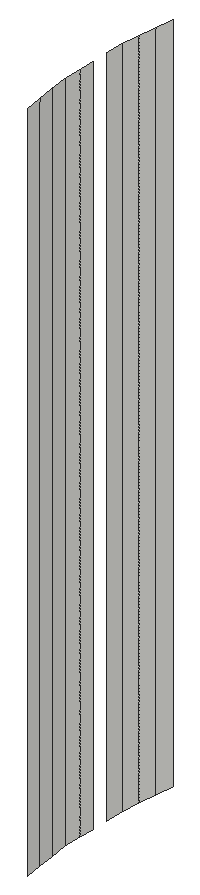
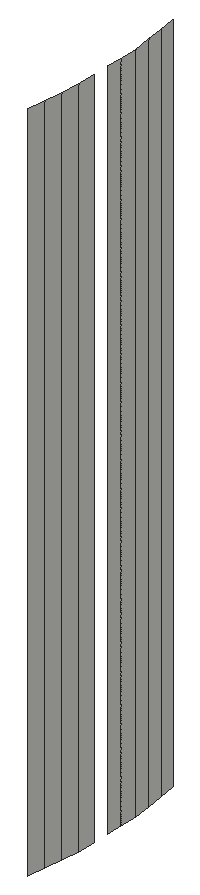
# SketchUp Ruby script. Lengths in inches.
U = 1.inch
M = Sketchup.active_model
def pt(a) = Geom::Point3d.new(a.map { |v| v * U })
def face(e, loops, mat)
  f = e.add_face(loops[0].map { |a| pt(a) })
  loops[1..].each { |l| e.add_face(l.map { |a| pt(a) }).erase! }
  f.material = f.back_material = mat if mat
  f
end
# faces: each face lists its corners as indices into pts; further lists are holes
def faces(e, pts, list, mat = nil) = list.each { |f| face(e, (f[0].is_a?(Array) ? f : [f]).map { |l| l.map { |i| pts[i] } }, mat) }
# xy, xz, yz: faces in a plane at the given z, y or x. An outline is a flat list of corners, or four numbers for a rectangle; further outlines are holes
def ring(l) = l.size == 4 ? [[l[0], l[1]], [l[2], l[1]], [l[2], l[3]], [l[0], l[3]]] : l.each_slice(2).to_a
def flat(e, list, mat, &to3) = list.each { |f| face(e, (f[0].is_a?(Array) ? f : [f]).map { |l| ring(l).map { |u, v| to3.(u, v) } }, mat) }
def xy(e, z, list, mat = nil) = flat(e, list, mat) { |x, y| [x, y, z] }
def xz(e, y, list, mat = nil) = flat(e, list, mat) { |x, z| [x, y, z] }
def yz(e, x, list, mat = nil) = flat(e, list, mat) { |y, z| [x, y, z] }
def lines(e, pts, list) = list.each { |a, b| e.add_line(pt(pts[a]), pt(pts[b])) }
# prism: a flat outline (further loops are holes) pulled along v
def prism(e, loops, v, mat = nil)
  f = face(e, loops, mat); d = Geom::Vector3d.new(v.map { |x| x * U })
  f.pushpull(f.normal.samedirection?(d) ? d.length : -d.length)
end
def box(e, o, s, mat = nil) = prism(e, [[o, [o[0] + s[0], o[1], o[2]], [o[0] + s[0], o[1] + s[1], o[2]], [o[0], o[1] + s[1], o[2]]]], [0, 0, s[2]], mat)
def at(x, y, z, deg = 0) = Geom::Transformation.translation(pt([x, y, z])) * Geom::Transformation.rotation(ORIGIN, Z_AXIS, deg.degrees)
def axes(o, x, y, z) = Geom::Transformation.new([*x, 0, *y, 0, *z, 0, *pt(o).to_a, 1])
def part(name) = M.definitions.add(name)
# library, detail: a bought-in or finely detailed component or shape, given as its bounding box
def library(name, o, s) = part(name).tap { |d| box(d.entities, o, s) }
def detail(e, o, s) = box(e.add_group.entities, o, s)
def put(e, d, t, mat = nil) = e.add_instance(d, t).tap { |i| i.material = mat if mat }
def group(e, t, mat = nil) = e.add_group.tap { |g| g.transformation = t; g.material = mat if mat }.entities
root = M.entities
yz(root,136.5,[[155.77,242,155.85,245],[155.85,242,155.92,245],[156,242,156.08,245]])
p = [[136.53,155.53,242],[136.52,155.61,242],[136.52,155.61,245],[136.53,155.53,245],[136.51,155.6875,242],[136.51,155.6875,245],
  [136.5,155.77,242],[136.5,155.77,245],[136.5,156.08,242],[136.51,156.16,242],[136.51,156.16,245],[136.5,156.08,245],
  [136.52,156.24,242],[136.52,156.24,245],[136.53,156.32,242],[136.53,156.32,245]]
faces(root,p,[[0,1,2,3],[1,4,5,2],[4,6,7,5],[8,9,10,11],[9,12,13,10],[12,14,15,13]])
